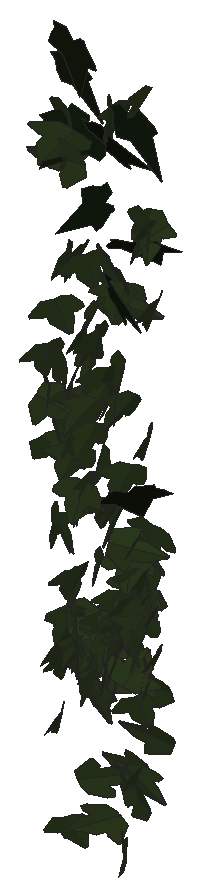
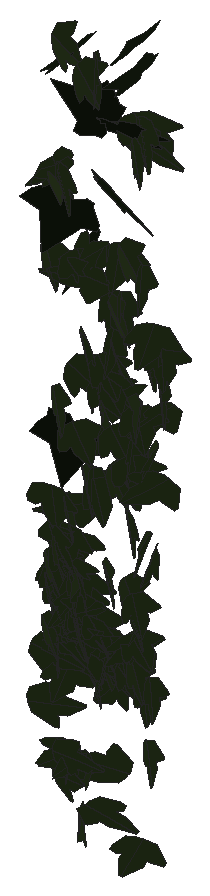
# SketchUp Ruby script. Lengths in inches.
U = 1.inch
M = Sketchup.active_model
def pt(a) = Geom::Point3d.new(a.map { |v| v * U })
def face(e, loops, mat)
  f = e.add_face(loops[0].map { |a| pt(a) })
  loops[1..].each { |l| e.add_face(l.map { |a| pt(a) }).erase! }
  f.material = f.back_material = mat if mat
  f
end
# faces: each face lists its corners as indices into pts; further lists are holes
def faces(e, pts, list, mat = nil) = list.each { |f| face(e, (f[0].is_a?(Array) ? f : [f]).map { |l| l.map { |i| pts[i] } }, mat) }
# xy, xz, yz: faces in a plane at the given z, y or x. An outline is a flat list of corners, or four numbers for a rectangle; further outlines are holes
def ring(l) = l.size == 4 ? [[l[0], l[1]], [l[2], l[1]], [l[2], l[3]], [l[0], l[3]]] : l.each_slice(2).to_a
def flat(e, list, mat, &to3) = list.each { |f| face(e, (f[0].is_a?(Array) ? f : [f]).map { |l| ring(l).map { |u, v| to3.(u, v) } }, mat) }
def xy(e, z, list, mat = nil) = flat(e, list, mat) { |x, y| [x, y, z] }
def xz(e, y, list, mat = nil) = flat(e, list, mat) { |x, z| [x, y, z] }
def yz(e, x, list, mat = nil) = flat(e, list, mat) { |y, z| [x, y, z] }
def lines(e, pts, list) = list.each { |a, b| e.add_line(pt(pts[a]), pt(pts[b])) }
# prism: a flat outline (further loops are holes) pulled along v
def prism(e, loops, v, mat = nil)
  f = face(e, loops, mat); d = Geom::Vector3d.new(v.map { |x| x * U })
  f.pushpull(f.normal.samedirection?(d) ? d.length : -d.length)
end
def box(e, o, s, mat = nil) = prism(e, [[o, [o[0] + s[0], o[1], o[2]], [o[0] + s[0], o[1] + s[1], o[2]], [o[0], o[1] + s[1], o[2]]]], [0, 0, s[2]], mat)
def at(x, y, z, deg = 0) = Geom::Transformation.translation(pt([x, y, z])) * Geom::Transformation.rotation(ORIGIN, Z_AXIS, deg.degrees)
def axes(o, x, y, z) = Geom::Transformation.new([*x, 0, *y, 0, *z, 0, *pt(o).to_a, 1])
def part(name) = M.definitions.add(name)
# library, detail: a bought-in or finely detailed component or shape, given as its bounding box
def library(name, o, s) = part(name).tap { |d| box(d.entities, o, s) }
def detail(e, o, s) = box(e.add_group.entities, o, s)
def put(e, d, t, mat = nil) = e.add_instance(d, t).tap { |i| i.material = mat if mat }
def group(e, t, mat = nil) = e.add_group.tap { |g| g.transformation = t; g.material = mat if mat }.entities
root = M.entities
M.materials.add("1026 AP 7946 SUNNY SIDE UP").color = [254, 231, 186]
M.materials.add("efeu1").color = [18, 25, 13]
M.materials.add("efeu2").color = [43, 57, 29]
c1 = part("ivyleaf_10")
p = [[0,0.5,-0.03],[-0.0625,2.02,-0.43],[-0.19,2.01,-0.46],[-0.54,1.05,-0.29],[-0.52,0.625,-0.18],[-0.83,0.76,-0.28],
  [-1.16,0.64,-0.33],[-1.15,0.33,-0.24],[-0.77,-0.39,0.02],[-0.3,-0.51,0.16],[0.04,-0.48,0.23],[-0.02,2.01,-0.4375],
  [-0.06,2.01,-0.43],[0.04,-0.49,0.23],[0.67,-0.49,0.14],[1.38,0.36,-0.2],[1.375,0.51,-0.24],[0.81,0.65,-0.19],
  [0.62,0.59,-0.15],[0.6,1.09,-0.28],[0.5,1.23,-0.31]]
faces(c1.entities,p,[[0,1,2,3,4,5,6,7,8,9,10],[11,12,0,13,14,15,16,17,18,19,20]],"efeu2")
c2 = part("ivyleaf_9")
p = [[1.54,2.16,1.25],[1.36,2.04,1.19],[-0.21,0.99,0.68],[-0.71,1.11,0.82],[-0.85,0.86,0.67],[-0.8,0.17,0.21],
  [-0.9,-0.01,0.1],[-0.67,-0.16,-0.02],[-0.08,-0.08,-0.05],[-0.03,-0.6,-0.4],[0.65,-0.88,-0.66],[0.83,-0.6,-0.49],
  [1.29,-0.42,-0.43],[1.8125,-0.07,-0.26],[1.21,0.44,0.15]]
faces(c2.entities,p,[[0,1,2,3,4,5,6,7,8,9,10,11,12,13,14]],"efeu1")
put(root,c1,axes([94.875,212.63,262.03],[0.11091,-0.09964,-0.20156],[-0.07635,0.19274,-0.11837],[0.33588,0.07671,0.03965]),"1026 AP 7946 SUNNY SIDE UP")
put(root,c1,axes([94.82,212.85,259.87],[0.04727,-0.10152,-0.20413],[0.02467,0.19984,-0.10216],[0.3484,-0.00038,0.03493]),"1026 AP 7946 SUNNY SIDE UP")
put(root,c1,axes([94.67,212.95,260.97],[-0.21375,-0.08063,-0.16071],[0.23552,0.04865,-0.16055],[0.14291,-0.20076,0.02421]),"1026 AP 7946 SUNNY SIDE UP")
put(root,c1,axes([94.79,212.96,263.03],[-0.20603,-0.17813,-0.07134],[0.10005,0.03723,-0.22577],[0.28277,-0.14296,0.0279]),"1026 AP 7946 SUNNY SIDE UP")
put(root,c1,axes([94.79,212.94,261.35],[-0.10546,0.21388,0.00706],[-0.00336,0.00524,-0.23089],[-0.33641,-0.0671,0.00009]),"1026 AP 7946 SUNNY SIDE UP")
put(root,c1,axes([94.85,212.875,258.04],[0.00414,-0.19667,-0.05433],[0.0162,0.05168,-0.20203],[0.31931,-0.00008,0.01096]),"1026 AP 7946 SUNNY SIDE UP")
put(root,c1,axes([94.91,212.96,265.85],[0.23307,-0.14192,-0.14244],[-0.05952,0.14827,-0.19887],[0.30492,0.13742,0.07006]),"1026 AP 7946 SUNNY SIDE UP")
put(root,c1,axes([94.89,212.62,262.58],[-0.11409,-0.21754,-0.0287],[0.02677,0.02236,-0.23593],[0.34356,-0.07398,0.00885]),"1026 AP 7946 SUNNY SIDE UP")
put(root,c1,axes([95.02,212.94,261.87],[0.0072,0.07591,0.22102],[-0.20721,0.17533,-0.06011],[-0.29096,-0.12298,0.04828]),"1026 AP 7946 SUNNY SIDE UP")
put(root,c1,axes([94.94,212.81,257.11],[0.0252,-0.18923,-0.08393],[-0.0133,0.07996,-0.19517],[0.32301,0.01805,-0.00149]),"1026 AP 7946 SUNNY SIDE UP")
put(root,c1,axes([94.91,212.97,263.8],[0.03515,-0.21492,-0.10042],[0.0389,0.0983,-0.21961],[0.36824,0.01013,0.03279]),"1026 AP 7946 SUNNY SIDE UP")
put(root,c1,axes([94.96,212.87,257.95],[-0.04201,-0.19828,-0.03988],[0.01307,0.0368,-0.20587],[0.31705,-0.02779,0.0032]),"1026 AP 7946 SUNNY SIDE UP")
put(root,c1,axes([94.81,212.65,261.79],[-0.04956,-0.15853,-0.17984],[0.21861,0.12876,-0.14632],[0.2982,-0.12074,0.07738]),"1026 AP 7946 SUNNY SIDE UP")
put(root,c1,axes([95.14,212.73,265.73],[-0.29498,-0.10258,0.14114],[-0.13082,-0.12391,-0.21278],[0.23602,-0.1969,0.05846]),"1026 AP 7946 SUNNY SIDE UP")
put(root,c1,axes([95.04,212.92,261.77],[-0.13885,-0.20808,0.0145],[0.00316,-0.01741,-0.2328],[0.32805,-0.08791,0.00838]),"1026 AP 7946 SUNNY SIDE UP")
put(root,c1,axes([95.27,212.65,265.45],[0.10246,-0.04411,-0.24964],[-0.35358,0.091,-0.07891],[0.15709,0.23359,-0.01478]),"1026 AP 7946 SUNNY SIDE UP")
put(root,c1,axes([95.04,212.96,258.27],[-0.00955,-0.20424,-0.01715],[-0.00708,0.01562,-0.21034],[0.32199,-0.00571,-0.00513]),"1026 AP 7946 SUNNY SIDE UP")
put(root,c1,axes([95.05,212.95,259.17],[-0.07402,-0.20554,-0.00202],[0.00397,0.00024,-0.21721],[0.32317,-0.04708,0.0022]),"1026 AP 7946 SUNNY SIDE UP")
put(root,c1,axes([95.08,212.91,258.62],[-0.10168,-0.18113,0.07939],[-0.00809,-0.08061,-0.19746],[0.31004,-0.0615,0.02088]),"1026 AP 7946 SUNNY SIDE UP")
put(root,c1,axes([95.09,212.87,258.57],[-0.09463,-0.18146,0.07993],[-0.01153,-0.08007,-0.19665],[0.31073,-0.05823,0.01705]),"1026 AP 7946 SUNNY SIDE UP")
put(root,c1,axes([95.0625,212.73,259.9375],[-0.1363,0.18226,0.08438],[-0.05596,0.07262,-0.20749],[-0.30849,-0.0937,0.00036]),"1026 AP 7946 SUNNY SIDE UP")
put(root,c1,axes([95.16,212.89,261.02],[-0.20213,-0.16038,0.08441],[-0.03114,-0.08857,-0.2088],[0.28213,-0.12468,0.03743]),"1026 AP 7946 SUNNY SIDE UP")
put(root,c1,axes([95.12,212.93,258.97],[0.14734,-0.1865,-0.01335],[-0.01278,0.00923,-0.21494],[0.29358,0.094,-0.00266]),"1026 AP 7946 SUNNY SIDE UP")
put(root,c1,axes([95.1,212.875,265.43],[0.08594,-0.23542,0.02469],[0.06457,-0.01614,-0.24627],[0.36666,0.05802,0.03759]),"1026 AP 7946 SUNNY SIDE UP")
put(root,c2,axes([95.25,212.97,265.77],[-0.36846,-0.07212,-0.00302],[0.01433,-0.02109,-0.2516],[0.11256,-0.23339,0.02216]),"1026 AP 7946 SUNNY SIDE UP")
put(root,c1,axes([95.18,212.54,262.5],[0.21714,-0.14388,-0.11921],[-0.0573,0.11942,-0.19848],[0.28379,0.1342,0.05114]),"1026 AP 7946 SUNNY SIDE UP")
put(root,c2,axes([94.95,213,266.62],[0.17422,-0.223,-0.00098],[0.00735,0.00197,-0.25646],[0.35056,0.11078,0.00586]),"1026 AP 7946 SUNNY SIDE UP")
put(root,c1,axes([95.16,212.91,260.29],[0.17891,-0.1786,-0.05029],[0.0083,0.05924,-0.21475],[0.2906,0.10827,0.0371]),"1026 AP 7946 SUNNY SIDE UP")
put(root,c1,axes([95.19,212.95,258.21],[-0.0344,-0.20069,0.03684],[-0.00138,-0.03701,-0.20817],[0.32085,-0.02168,0.00305]),"1026 AP 7946 SUNNY SIDE UP")
put(root,c1,axes([95.18,212.92,258.21],[-0.03672,-0.16774,0.11451],[0.01346,-0.11358,-0.1739],[0.31695,-0.01461,0.02066]),"1026 AP 7946 SUNNY SIDE UP")
put(root,c1,axes([95.1875,212.95,263.99],[0.06339,-0.22614,0.06233],[-0.00042,-0.06274,-0.23674],[0.36862,0.03882,-0.01099]),"1026 AP 7946 SUNNY SIDE UP")
put(root,c1,axes([95.15,212.85,261.28],[0.03346,-0.20553,-0.08471],[0.05769,0.08359,-0.20794],[0.34258,0.006,0.04329]),"1026 AP 7946 SUNNY SIDE UP")
put(root,c2,axes([95.03,212.98,266.97],[0.02774,-0.23217,0.09478],[0.00615,-0.09328,-0.2404],[0.39341,0.01783,-0.00293]),"1026 AP 7946 SUNNY SIDE UP")
put(root,c1,axes([95.125,212.96,258.67],[0.05461,0.20022,0.00144],[-0.00136,0.00042,-0.20934],[-0.31482,0.03473,0.00116]),"1026 AP 7946 SUNNY SIDE UP")
put(root,c1,axes([95.22,212.86,259.31],[-0.00684,-0.20926,0.03367],[0.00162,-0.0339,-0.21581],[0.33332,-0.00413,0.00174]),"1026 AP 7946 SUNNY SIDE UP")
put(root,c1,axes([95.17,212.73,255.65],[-0.2313,-0.12008,-0.07986],[0.10882,0.03637,-0.19484],[0.19597,-0.16192,0.01394]),"1026 AP 7946 SUNNY SIDE UP")
put(root,c1,axes([95.21,212.95,258.47],[0.02973,0.19828,-0.03877],[-0.02581,-0.03729,-0.205],[-0.31663,0.02166,0.01307]),"1026 AP 7946 SUNNY SIDE UP")
put(root,c1,axes([95.37,212.94,261.4],[-0.14184,-0.18723,0.08494],[-0.0011,-0.09096,-0.21138],[0.32235,-0.08269,0.03666]),"1026 AP 7946 SUNNY SIDE UP")
put(root,c1,axes([95.18,212.86,258.11],[0.04979,-0.04369,0.20623],[0.20704,-0.15119,-0.05626],[0.24735,0.13534,0.00558]),"1026 AP 7946 SUNNY SIDE UP")
put(root,c1,axes([95.34,212.89,263.92],[-0.16931,-0.20442,-0.05215],[0.07403,0.03073,-0.23625],[0.32232,-0.11444,0.02686]),"1026 AP 7946 SUNNY SIDE UP")
put(root,c1,axes([95.38,212.93,263.13],[0.13998,-0.21403,0.02669],[-0.00048,-0.02947,-0.23868],[0.33923,0.08827,-0.01135]),"1026 AP 7946 SUNNY SIDE UP")
put(root,c1,axes([95.45,212.79,261.84],[-0.09904,-0.15774,0.15177],[-0.02461,-0.15064,-0.1729],[0.33945,-0.05694,0.03174]),"1026 AP 7946 SUNNY SIDE UP")
put(root,c1,axes([95.4,212.9375,262.73],[0.01075,-0.19275,-0.13434],[0.03836,0.12924,-0.19639],[0.36294,-0.00795,0.02474]),"1026 AP 7946 SUNNY SIDE UP")
put(root,c1,axes([95.32,212.94,262.5],[0.22723,-0.1362,0.12066],[0.12237,-0.08911,-0.20484],[0.25545,0.16384,-0.00921]),"1026 AP 7946 SUNNY SIDE UP")
put(root,c2,axes([95.58,212.91,264.8125],[-0.32696,0.11146,-0.05198],[0.05171,-0.0462,-0.24199],[-0.18573,-0.20907,0.02413]),"1026 AP 7946 SUNNY SIDE UP")
put(root,c1,axes([95.39,212.68,260.64],[0.34397,-0.0276,0.00497],[0.00351,-0.02191,-0.22619],[0.04396,0.21771,-0.02083]),"1026 AP 7946 SUNNY SIDE UP")
put(root,c1,axes([95.46,212.84,260.78],[0.02358,-0.21367,0.05155],[0.01258,-0.0508,-0.22092],[0.34528,0.01644,0.00453]),"1026 AP 7946 SUNNY SIDE UP")
put(root,c1,axes([95.46,212.98,259.49],[0.12875,-0.1919,-0.03618],[0.00123,0.03723,-0.21415],[0.30644,0.08048,0.01606]),"1026 AP 7946 SUNNY SIDE UP")
put(root,c1,axes([95.41,212.95,258.52],[0.27124,0.1123,-0.01783],[-0.0097,-0.02331,-0.21153],[-0.17855,0.17186,-0.01559]),"1026 AP 7946 SUNNY SIDE UP")
put(root,c1,axes([95.49,212.61,263.05],[0.03067,-0.22822,-0.09039],[0.00102,0.08677,-0.23533],[0.38372,0.01801,0.00785]),"1026 AP 7946 SUNNY SIDE UP")
put(root,c1,axes([95.54,212.94,262.04],[-0.14253,-0.1857,0.09745],[-0.00345,-0.10341,-0.20958],[0.32843,-0.08167,0.04009]),"1026 AP 7946 SUNNY SIDE UP")
put(root,c1,axes([95.45,212.92,258.36],[-0.2822,0.05209,-0.08284],[0.09213,-0.07618,-0.18531],[-0.1197,-0.18144,0.05268]),"1026 AP 7946 SUNNY SIDE UP")
put(root,c1,axes([95.51,213,258.16],[-0.15373,0.17493,0.0325],[-0.03628,0.02207,-0.20609],[-0.27685,-0.10003,0.00896]),"1026 AP 7946 SUNNY SIDE UP")
put(root,c1,axes([95.58,212.97,258.22],[-0.07032,-0.11719,0.16341],[-0.03469,-0.15933,-0.12807],[0.309,-0.04455,0.02281]),"1026 AP 7946 SUNNY SIDE UP")
put(root,c1,axes([95.57,212.92,262.31],[-0.07713,-0.21864,0.04935],[-0.00991,-0.04895,-0.23108],[0.35223,-0.04925,0.00431]),"1026 AP 7946 SUNNY SIDE UP")
put(root,c1,axes([95.55,212.88,258.37],[0.12005,-0.19199,-0.00308],[-0.00775,0.00008,-0.2128],[0.30179,0.07637,-0.00424]),"1026 AP 7946 SUNNY SIDE UP")
put(root,c1,axes([95.35,212.84,258.02],[0.13757,-0.03837,0.19171],[0.26422,-0.08051,-0.09885],[0.14017,0.18943,-0.00183]),"1026 AP 7946 SUNNY SIDE UP")
put(root,c1,axes([95.64,212.94,258.74],[-0.12055,-0.19032,0.03684],[-0.01725,-0.03529,-0.21156],[0.30432,-0.07739,0.0026]),"1026 AP 7946 SUNNY SIDE UP")
put(root,c1,axes([95.57,212.96,258.57],[-0.26949,-0.10917,-0.03468],[0.08425,-0.02441,-0.20337],[0.15833,-0.17283,0.04919]),"1026 AP 7946 SUNNY SIDE UP")
put(root,c1,axes([95.62,212.68,257.98],[0.03188,-0.1864,0.08074],[0.02608,-0.07803,-0.19346],[0.31753,0.02513,0.00778]),"1026 AP 7946 SUNNY SIDE UP")
put(root,c1,axes([95.66,212.9,258.18],[-0.03373,-0.17784,0.10114],[0.00355,-0.09993,-0.18467],[0.32016,-0.01763,0.0127]),"1026 AP 7946 SUNNY SIDE UP")
put(root,c1,axes([95.66,212.66,263.03],[-0.03756,-0.23195,-0.05627],[0.02076,0.0522,-0.23978],[0.37364,-0.02621,0.00766]),"1026 AP 7946 SUNNY SIDE UP")
put(root,c1,axes([95.7,212.89,262.04],[0.09892,-0.20116,-0.0897],[-0.03359,0.08334,-0.21661],[0.34232,0.06631,0.00467]),"1026 AP 7946 SUNNY SIDE UP")
put(root,c1,axes([95.57,212.71,257.78],[-0.2755,0.07203,-0.09651],[0.11776,-0.06285,-0.1936],[-0.1444,-0.18868,0.02625]),"1026 AP 7946 SUNNY SIDE UP")
put(root,c1,axes([95.83,212.93,263.7],[-0.23953,0.10338,-0.15412],[-0.17889,0.09904,0.18969],[0.22403,0.18961,-0.01331]),"1026 AP 7946 SUNNY SIDE UP")
put(root,c1,axes([95.71,212.87,260.5],[-0.08348,-0.21241,0.00316],[0.00155,-0.00465,-0.22557],[0.33405,-0.05306,0.00183]),"1026 AP 7946 SUNNY SIDE UP")
put(root,c1,axes([95.84,212.72,255.9375],[0.19913,0.02327,-0.17259],[-0.25325,-0.04785,-0.13245],[-0.08188,0.20459,-0.01007]),"1026 AP 7946 SUNNY SIDE UP")
put(root,c1,axes([95.63,212.99,258.54],[0.20372,0.15326,0.04023],[0.04768,0.02432,-0.20646],[-0.24373,0.13286,-0.00677]),"1026 AP 7946 SUNNY SIDE UP")
put(root,c1,axes([95.75,212.71,261.27],[-0.05051,0.14915,-0.17003],[-0.03384,-0.16889,-0.15313],[-0.34914,-0.00521,0.03944]),"1026 AP 7946 SUNNY SIDE UP")
put(root,c1,axes([95.74,212.78,258.45],[0.10414,0.17407,-0.08325],[-0.03312,-0.07943,-0.19216],[-0.3006,0.06905,-0.00767]),"1026 AP 7946 SUNNY SIDE UP")
put(root,c1,axes([95.79,212.81,260.6],[0.01915,-0.208,-0.0763],[0.02937,0.0737,-0.21305],[0.34531,0.00526,0.02235]),"1026 AP 7946 SUNNY SIDE UP")
put(root,c1,axes([95.75,212.98,258.7],[0.31828,-0.0398,-0.00354],[-0.00479,0.00116,-0.21251],[0.0626,0.20244,0.00175]),"1026 AP 7946 SUNNY SIDE UP")
put(root,c1,axes([95.76,212.99,258.77],[0.18524,0.16192,-0.04767],[-0.02788,-0.04536,-0.20618],[-0.26373,0.11853,-0.01169]),"1026 AP 7946 SUNNY SIDE UP")
put(root,c1,axes([95.83,212.98,266.29],[0.00384,-0.23401,0.08431],[0.01501,-0.08302,-0.24143],[0.39022,0.00549,0.00846]),"1026 AP 7946 SUNNY SIDE UP")
put(root,c1,axes([95.64,212.58,256.5],[-0.08327,-0.04847,0.21431],[0.18481,0.17268,0.07319],[-0.28095,0.12796,-0.01538]),"1026 AP 7946 SUNNY SIDE UP")
put(root,c1,axes([95.85,212.9,260.65],[0.09068,-0.20265,-0.06666],[-0.01574,0.06319,-0.21655],[0.33358,0.05807,0.0079]),"1026 AP 7946 SUNNY SIDE UP")
put(root,c1,axes([95.84,212.99,258.79],[-0.09761,-0.1924,0.03751],[0.01902,-0.04303,-0.20701],[0.30764,-0.05839,0.0247]),"1026 AP 7946 SUNNY SIDE UP")
put(root,c1,axes([95.84,212.59,258.14],[0.11792,-0.16287,-0.11062],[-0.00745,0.11253,-0.18014],[0.30587,0.06553,0.03826]),"1026 AP 7946 SUNNY SIDE UP")
put(root,c1,axes([95.85,212.75,257.86],[0.14986,-0.17051,-0.06511],[-0.023,0.06285,-0.2001],[0.28448,0.0949,0.01812]),"1026 AP 7946 SUNNY SIDE UP")
put(root,c1,axes([95.82,212.8125,262.07],[0.18491,-0.17967,-0.08108],[0.01716,0.0965,-0.21235],[0.30731,0.10272,0.06064]),"1026 AP 7946 SUNNY SIDE UP")
put(root,c1,axes([95.82,212.74,266.33],[0.13962,-0.2156,-0.08953],[0.03113,0.09845,-0.2335],[0.36347,0.07439,0.05439]),"1026 AP 7946 SUNNY SIDE UP")
put(root,c1,axes([95.92,212.96,259.12],[0.05194,-0.02207,0.20996],[-0.16129,0.1771,0.0379],[-0.27931,-0.10637,0.01716]),"1026 AP 7946 SUNNY SIDE UP")
put(root,c1,axes([95.75,212.96,258.9],[0.11708,0.14123,0.13647],[0.04487,0.13153,-0.16118],[-0.30028,0.07472,0.02913]),"1026 AP 7946 SUNNY SIDE UP")
put(root,c1,axes([95.875,213.02,258.6],[0.09376,-0.19335,-0.01755],[-0.00272,0.01614,-0.20833],[0.30505,0.05958,0.00353]),"1026 AP 7946 SUNNY SIDE UP")
put(root,c1,axes([95.86,212.91,262.52],[0.19452,-0.19212,-0.0325],[0.00617,0.03855,-0.23388],[0.3058,0.12143,0.02539]),"1026 AP 7946 SUNNY SIDE UP")
put(root,c2,axes([95.58,212.92,265.73],[0.11667,-0.10766,0.21408],[0.2304,-0.14944,-0.13414],[0.28805,0.16314,0.02058]),"1026 AP 7946 SUNNY SIDE UP")
put(root,c1,axes([95.92,212.92,263.66],[-0.22054,-0.18055,0.06453],[0.00543,-0.0813,-0.23015],[0.30099,-0.13083,0.05144]),"1026 AP 7946 SUNNY SIDE UP")
put(root,c1,axes([95.9,212.9,259.14],[-0.22213,-0.15575,0.00454],[0.02388,-0.02086,-0.21518],[0.24388,-0.13982,0.0252]),"1026 AP 7946 SUNNY SIDE UP")
put(root,c1,axes([95.89,212.78,258.76],[-0.06776,0.1744,-0.10164],[-0.03919,-0.10577,-0.18022],[-0.3134,-0.02448,0.04451]),"1026 AP 7946 SUNNY SIDE UP")
put(root,c1,axes([95.92,212.95,259.19],[0.14668,-0.17892,-0.05121],[-0.01661,0.04929,-0.20714],[0.29109,0.09297,0.01398]),"1026 AP 7946 SUNNY SIDE UP")
put(root,c1,axes([95.9375,212.87,258.57],[-0.0353,-0.18473,0.09335],[0.01184,-0.09288,-0.19147],[0.32405,-0.01673,0.01717]),"1026 AP 7946 SUNNY SIDE UP")
put(root,c1,axes([95.96,212.9,258.81],[0.00059,-0.20447,0.04034],[-0.00381,-0.04032,-0.21086],[0.32768,-0.0001,-0.00252]),"1026 AP 7946 SUNNY SIDE UP")
put(root,c1,axes([95.89,212.84,256.59],[-0.17092,0.1539,-0.07522],[0.05134,-0.06724,-0.19415],[-0.26348,-0.11293,0.01096]),"1026 AP 7946 SUNNY SIDE UP")
put(root,c1,axes([95.97,212.95,258.91],[0.06903,-0.19299,-0.06097],[-0.00598,0.05864,-0.20334],[0.31684,0.04315,0.00945]),"1026 AP 7946 SUNNY SIDE UP")
put(root,c1,axes([96,212.93,259],[-0.27079,-0.11444,0.01538],[-0.00587,-0.02244,-0.21246],[0.18151,-0.17145,0.01608]),"1026 AP 7946 SUNNY SIDE UP")
put(root,c1,axes([96.01,212.89,262.07],[-0.04599,-0.1762,0.14504],[-0.02356,-0.14115,-0.18471],[0.35484,-0.03221,0.00654]),"1026 AP 7946 SUNNY SIDE UP")
put(root,c1,axes([96.1875,212.91,256.66],[-0.00384,-0.0098,-0.21014],[-0.30237,0.06864,-0.00063],[0.10787,0.19205,-0.00923]),"1026 AP 7946 SUNNY SIDE UP")
put(root,c1,axes([95.96,212.71,260.46],[0.14455,-0.19766,0.06215],[0.02864,-0.05926,-0.22476],[0.32421,0.09336,-0.00786]),"1026 AP 7946 SUNNY SIDE UP")
put(root,c2,axes([95.9,212.6875,263.76],[0.26004,-0.10504,-0.14742],[-0.1831,0.08234,-0.20126],[0.20966,0.20218,0.00707]),"1026 AP 7946 SUNNY SIDE UP")
put(root,c1,axes([96.02,212.61,258.45],[0.11243,-0.18611,-0.06617],[-0.01262,0.06441,-0.20445],[0.30879,0.07039,0.01574]),"1026 AP 7946 SUNNY SIDE UP")
put(root,c1,axes([96.03,212.86,259.15],[-0.02576,-0.20678,-0.04546],[0.00237,0.04297,-0.21343],[0.33207,-0.01635,-0.002]),"1026 AP 7946 SUNNY SIDE UP")
put(root,c1,axes([95.73,212.92,263.46],[-0.07058,-0.02692,-0.23755],[0.36311,0.01736,-0.04833],[0.03504,-0.23412,0.02234]),"1026 AP 7946 SUNNY SIDE UP")
put(root,c1,axes([95.97,212.98,258.91],[-0.09763,-0.14763,-0.13601],[0.14683,0.09923,-0.15998],[0.27363,-0.10592,0.03732]),"1026 AP 7946 SUNNY SIDE UP")
put(root,c1,axes([96.11,212.77,261.125],[-0.17655,-0.17953,0.07261],[-0.01326,-0.07806,-0.21602],[0.30357,-0.10782,0.03279]),"1026 AP 7946 SUNNY SIDE UP")
put(root,c1,axes([96.01,212.8125,258.69],[-0.25688,0.10919,-0.06712],[0.0676,-0.05346,-0.20174],[-0.18869,-0.1678,0.0191]),"1026 AP 7946 SUNNY SIDE UP")
put(root,c1,axes([96.11,212.96,259.35],[0.29269,0.04264,-0.08991],[-0.12749,-0.03661,-0.19625],[-0.08472,0.20241,-0.01528]),"1026 AP 7946 SUNNY SIDE UP")
put(root,c1,axes([96.15,212.87,258.12],[0.27267,0.02688,-0.11269],[-0.16834,-0.02402,-0.18081],[-0.05583,0.2037,-0.00522]),"1026 AP 7946 SUNNY SIDE UP")
put(root,c1,axes([96.02,212.89,259.74],[0.31496,0.07166,0.00417],[0.01372,-0.01362,-0.21864],[-0.11199,0.19988,-0.01507]),"1026 AP 7946 SUNNY SIDE UP")
put(root,c1,axes([96.13,212.96,259.79],[-0.33623,0.01714,0.01048],[-0.01844,-0.02092,-0.21997],[-0.02524,-0.21304,0.02117]),"1026 AP 7946 SUNNY SIDE UP")
put(root,c1,axes([96.15,212.97,259.53],[-0.11411,-0.19238,0.0454],[-0.02023,-0.04341,-0.21205],[0.31006,-0.07363,0.00288]),"1026 AP 7946 SUNNY SIDE UP")
put(root,c2,axes([96.09,212.92,264.4],[0.28689,0.1574,-0.01334],[-0.0484,0.01466,-0.24607],[-0.24369,0.18239,0.03317]),"1026 AP 7946 SUNNY SIDE UP")
put(root,c1,axes([96.17,212.98,259.23],[-0.21315,-0.15705,0.01632],[0.00205,-0.02317,-0.21322],[0.24833,-0.1346,0.01577]),"1026 AP 7946 SUNNY SIDE UP")
put(root,c1,axes([96.18,212.85,260.14],[0.0738,-0.19802,-0.07848],[-0.02231,0.07376,-0.2092],[0.33224,0.04894,0.00338]),"1026 AP 7946 SUNNY SIDE UP")
put(root,c1,axes([96.23,212.52,255.59],[-0.00142,-0.02722,-0.23115],[-0.06589,0.22035,-0.0261],[0.34899,0.04149,-0.00587]),"1026 AP 7946 SUNNY SIDE UP")
put(root,c1,axes([96.34,212.78,256.27],[-0.06264,0.03368,-0.20733],[-0.21097,0.15042,0.05412],[0.24213,0.13978,-0.00648]),"1026 AP 7946 SUNNY SIDE UP")
put(root,c1,axes([96.1875,212.71,256.48],[0.03151,0.0029,0.22045],[-0.08281,0.20837,0.00339],[-0.32613,-0.05263,0.02044]),"1026 AP 7946 SUNNY SIDE UP")
put(root,c1,axes([96.27,212.82,258.9375],[-0.22884,-0.12947,0.07343],[-0.0458,-0.07397,-0.19808],[0.22841,-0.14455,0.03385]),"1026 AP 7946 SUNNY SIDE UP")
put(root,c1,axes([96.22,213.03,258.8],[0.13363,-0.1857,0.0036],[-0.00467,-0.00636,-0.21035],[0.29204,0.08487,-0.00501]),"1026 AP 7946 SUNNY SIDE UP")
put(root,c1,axes([96.21,212.96,266.61],[0.07602,-0.19842,0.14851],[0.04051,-0.14317,-0.2111],[0.38456,0.0543,-0.00712]),"1026 AP 7946 SUNNY SIDE UP")
put(root,c1,axes([96.24,212.91,264.76],[0.24682,-0.1674,-0.08549],[-0.0381,0.08802,-0.23226],[0.29064,0.15369,0.04216]),"1026 AP 7946 SUNNY SIDE UP")
put(root,c1,axes([96.33,212.95,259.69],[0.19143,-0.10465,-0.14199],[-0.15531,0.09547,-0.16471],[0.22253,0.15665,0.00719]),"1026 AP 7946 SUNNY SIDE UP")
put(root,c1,axes([96.24,212.96,259.58],[0.04196,-0.20627,-0.02442],[0.00644,0.02324,-0.21401],[0.3262,0.02607,0.00737]),"1026 AP 7946 SUNNY SIDE UP")
put(root,c1,axes([96.28,212.71,258.57],[0.14685,-0.18055,-0.04505],[-0.02237,0.0407,-0.20909],[0.29088,0.09428,0.00667]),"1026 AP 7946 SUNNY SIDE UP")
put(root,c1,axes([96.29,212.93,261.62],[0.05983,-0.21274,-0.07007],[-0.01231,0.06646,-0.22222],[0.3504,0.03866,0.00416]),"1026 AP 7946 SUNNY SIDE UP")
put(root,c1,axes([96.23,212.8,257.76],[-0.20307,-0.14642,-0.06805],[0.09672,0.03207,-0.19947],[0.23274,-0.14108,0.02352]),"1026 AP 7946 SUNNY SIDE UP")
put(root,c1,axes([96.36,212.96,260.25],[-0.32852,0.03167,0.04219],[-0.07186,-0.03433,-0.21395],[-0.03779,-0.21008,0.04004]),"1026 AP 7946 SUNNY SIDE UP")
put(root,c1,axes([96.07,212.66,260.07],[-0.01837,-0.08576,-0.22248],[0.31094,0.10902,-0.05511],[0.1905,-0.18622,0.0685]),"1026 AP 7946 SUNNY SIDE UP")
put(root,c1,axes([96.18,212.67,258.14],[0.27323,0.07838,-0.10954],[0.13032,0.07305,0.19462],[0.16247,-0.19042,0.02811]),"1026 AP 7946 SUNNY SIDE UP")
put(root,c1,axes([96.33,213.01,259.36],[0.06806,-0.20377,-0.00368],[-0.00637,0.0016,-0.21457],[0.32037,0.04332,-0.00349]),"1026 AP 7946 SUNNY SIDE UP")
put(root,c1,axes([96.31,212.93,264.7],[0.10073,-0.20988,0.10679],[0.02831,-0.10397,-0.22634],[0.36782,0.06548,-0.01182]),"1026 AP 7946 SUNNY SIDE UP")
put(root,c1,axes([96.16,212.84,256.66],[-0.24052,0.00219,-0.14165],[0.21345,-0.03051,-0.15625],[-0.03461,-0.20341,0.02069]),"1026 AP 7946 SUNNY SIDE UP")
put(root,c1,axes([96.54,212.88,258.01],[0.06379,0.04157,-0.20259],[-0.30725,0.05612,-0.02894],[0.07559,0.19303,0.05332]),"1026 AP 7946 SUNNY SIDE UP")
put(root,c2,axes([96.32,212.53,260.98],[0.18573,0.21202,-0.01766],[0.00181,-0.02162,-0.24987],[-0.33462,0.11756,-0.01115]),"1026 AP 7946 SUNNY SIDE UP")
put(root,c1,axes([96.31,212.87,259.2],[-0.16112,-0.1795,-0.0364],[0.07733,0.0108,-0.20946],[0.27676,-0.10752,0.03734]),"1026 AP 7946 SUNNY SIDE UP")
put(root,c1,axes([96.57,212.89,257.25],[-0.08232,0.0333,-0.20399],[-0.31539,0.00424,0.05534],[0.01991,0.20496,0.03323]),"1026 AP 7946 SUNNY SIDE UP")
put(root,c1,axes([96.35,212.91,264.86],[0.07628,0.21799,-0.1005],[-0.09606,-0.08619,-0.22732],[-0.36386,0.06845,0.03894]),"1026 AP 7946 SUNNY SIDE UP")
put(root,c1,axes([96.37,212.98,259.09],[0.06507,-0.1938,-0.06334],[-0.00963,0.06041,-0.20369],[0.31904,0.04135,0.00677]),"1026 AP 7946 SUNNY SIDE UP")
put(root,c1,axes([96.37,212.75,258.32],[0.14659,-0.16768,-0.06767],[-0.00685,0.0708,-0.19496],[0.28254,0.08871,0.03039]),"1026 AP 7946 SUNNY SIDE UP")
put(root,c1,axes([96.4,212.78,258.11],[0.0905,-0.16488,-0.11658],[-0.02175,0.11323,-0.17801],[0.31286,0.05557,0.02135]),"1026 AP 7946 SUNNY SIDE UP")
put(root,c2,axes([96.1875,212.73,266.38],[0.13784,-0.24606,-0.02437],[-0.00621,0.02221,-0.26894],[0.38844,0.08767,0.00434]),"1026 AP 7946 SUNNY SIDE UP")
put(root,c1,axes([96.2,212.97,259.43],[0.0736,-0.02945,0.20954],[0.24145,-0.1339,-0.05711],[0.21518,0.16032,-0.00758]),"1026 AP 7946 SUNNY SIDE UP")
put(root,c1,axes([96.41,212.93,263.625],[0.02712,-0.23457,-0.03263],[-0.00488,0.03019,-0.24213],[0.37188,0.01751,-0.0008]),"1026 AP 7946 SUNNY SIDE UP")
put(root,c1,axes([96.33,212.92,264.77],[0.11811,0.22214,-0.06691],[-0.01874,-0.0658,-0.24177],[-0.364,0.07547,-0.00926]),"1026 AP 7946 SUNNY SIDE UP")
put(root,c1,axes([96.41,212.96,258.42],[0.05414,-0.20174,-0.01439],[-0.0114,0.01177,-0.2107],[0.31764,0.0348,-0.00511]),"1026 AP 7946 SUNNY SIDE UP")
